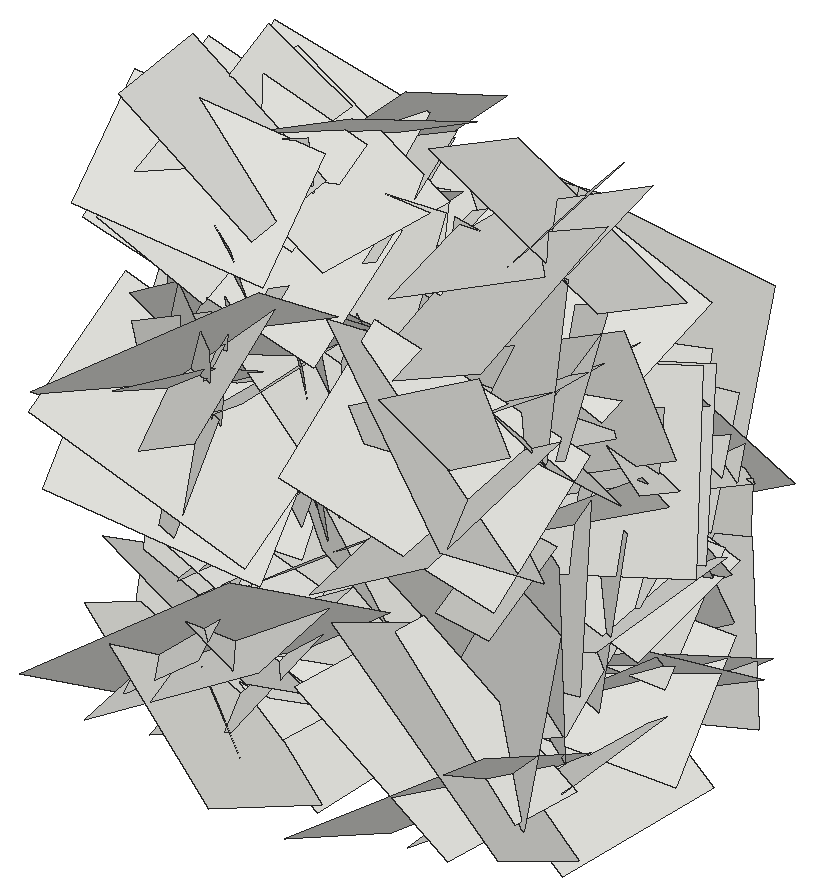
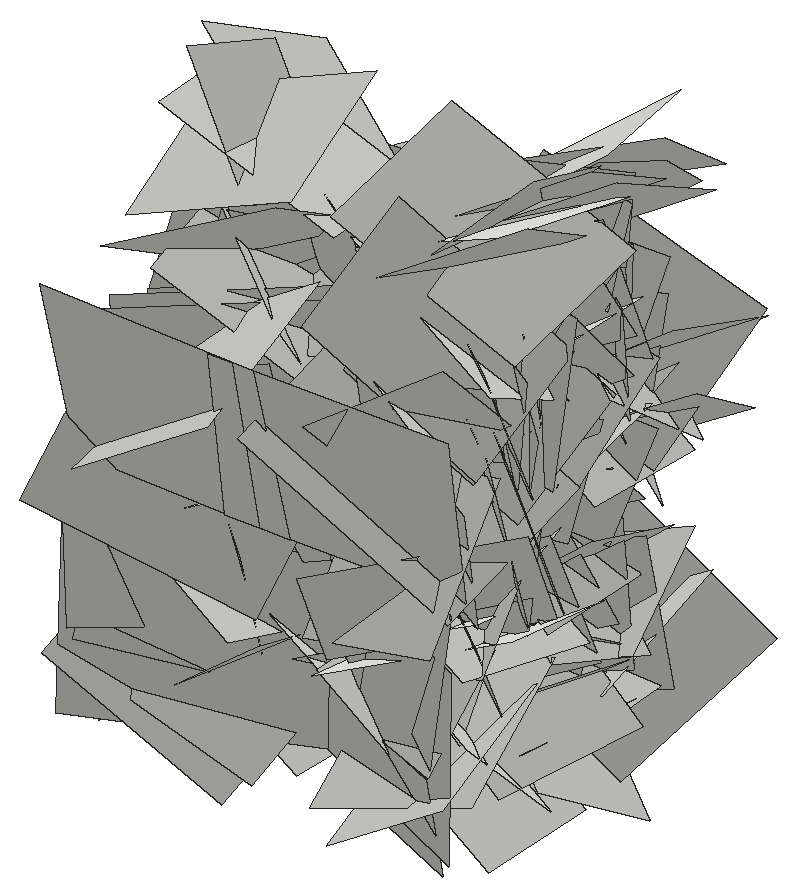
# SketchUp Ruby script. Lengths in inches.
U = 1.inch
M = Sketchup.active_model
def pt(a) = Geom::Point3d.new(a.map { |v| v * U })
def face(e, loops, mat)
  f = e.add_face(loops[0].map { |a| pt(a) })
  loops[1..].each { |l| e.add_face(l.map { |a| pt(a) }).erase! }
  f.material = f.back_material = mat if mat
  f
end
# faces: each face lists its corners as indices into pts; further lists are holes
def faces(e, pts, list, mat = nil) = list.each { |f| face(e, (f[0].is_a?(Array) ? f : [f]).map { |l| l.map { |i| pts[i] } }, mat) }
# xy, xz, yz: faces in a plane at the given z, y or x. An outline is a flat list of corners, or four numbers for a rectangle; further outlines are holes
def ring(l) = l.size == 4 ? [[l[0], l[1]], [l[2], l[1]], [l[2], l[3]], [l[0], l[3]]] : l.each_slice(2).to_a
def flat(e, list, mat, &to3) = list.each { |f| face(e, (f[0].is_a?(Array) ? f : [f]).map { |l| ring(l).map { |u, v| to3.(u, v) } }, mat) }
def xy(e, z, list, mat = nil) = flat(e, list, mat) { |x, y| [x, y, z] }
def xz(e, y, list, mat = nil) = flat(e, list, mat) { |x, z| [x, y, z] }
def yz(e, x, list, mat = nil) = flat(e, list, mat) { |y, z| [x, y, z] }
def lines(e, pts, list) = list.each { |a, b| e.add_line(pt(pts[a]), pt(pts[b])) }
# prism: a flat outline (further loops are holes) pulled along v
def prism(e, loops, v, mat = nil)
  f = face(e, loops, mat); d = Geom::Vector3d.new(v.map { |x| x * U })
  f.pushpull(f.normal.samedirection?(d) ? d.length : -d.length)
end
def box(e, o, s, mat = nil) = prism(e, [[o, [o[0] + s[0], o[1], o[2]], [o[0] + s[0], o[1] + s[1], o[2]], [o[0], o[1] + s[1], o[2]]]], [0, 0, s[2]], mat)
def at(x, y, z, deg = 0) = Geom::Transformation.translation(pt([x, y, z])) * Geom::Transformation.rotation(ORIGIN, Z_AXIS, deg.degrees)
def axes(o, x, y, z) = Geom::Transformation.new([*x, 0, *y, 0, *z, 0, *pt(o).to_a, 1])
def part(name) = M.definitions.add(name)
# library, detail: a bought-in or finely detailed component or shape, given as its bounding box
def library(name, o, s) = part(name).tap { |d| box(d.entities, o, s) }
def detail(e, o, s) = box(e.add_group.entities, o, s)
def put(e, d, t, mat = nil) = e.add_instance(d, t).tap { |i| i.material = mat if mat }
def group(e, t, mat = nil) = e.add_group.tap { |g| g.transformation = t; g.material = mat if mat }.entities
root = M.entities
c1 = part("Component\#6")
p = [[0.01,0,0],[0,3.24,4.54],[4.32,3.24,4.54],[4.33,0,0]]
faces(c1.entities,p,[[0,1,2,3]])
put(root,c1,axes([414.68,209.1,25.86],[0.06992,-0.92649,-0.30548],[0.11921,-0.29692,0.92479],[-1.02719,-0.09753,0.08653]))
put(root,c1,axes([410.71,209.1,25.86],[-0.06992,-0.92649,-0.30548],[-0.11921,-0.29692,0.92479],[1.02719,-0.09753,0.08653]))
put(root,c1,axes([410.71,210.17,27.25],[0.0389,-0.19659,0.74237],[0.03773,0.74285,0.19496],[0.81316,-0.02506,-0.04456]))
put(root,c1,axes([414.68,202.89,32.22],[0.0211,0.0618,0.84202],[0.01452,0.84212,-0.06213],[-0.89482,0.01512,0.01885]))
put(root,c1,axes([410.71,209.27,26.87],[0.02942,-0.98917,0.00062],[-0.2303,-0.00549,0.9654],[1.02292,0.02721,0.21733]))
put(root,c1,axes([410.71,208.86,27.22],[-0.22907,0.58895,0.94038],[-0.09031,0.94642,-0.61231],[1.17269,0.18793,0.13653]))
put(root,c1,axes([410.71,209.72,22.08],[-0.18138,-0.91546,-0.54155],[-0.07402,-0.53767,0.93095],[1.12504,-0.18297,-0.02606]))
put(root,c1,axes([410.71,200.125,30.08],[-0.25415,0.9144,0.59243],[-0.00684,0.60541,-0.93704],[1.1549,0.20481,0.12483]))
put(root,c1,axes([414.68,207.43,34.16],[-0.11276,0.04323,0.70746],[0.03845,0.71477,-0.03823],[-0.75032,0.03013,-0.10828]))
put(root,c1,axes([410.71,204.07,39.0625],[-0.02986,0.79051,0.40956],[0.00815,0.40997,-0.79076],[0.94369,0.02147,0.01979]))
put(root,c1,axes([414.68,209.14,33.82],[-0.16184,0.36707,0.52708],[0.01835,0.54392,-0.37378],[-0.68059,-0.07262,-0.13541]))
put(root,c1,axes([410.71,210.92,34.25],[0.13403,0.53039,0.57824],[-0.04314,0.58935,-0.53168],[0.83061,-0.05497,-0.12092]))
put(root,c1,axes([414.68,209.37,33.75],[0.00852,0.3462,-0.76666],[0.09329,-0.76284,-0.34355],[-0.88678,-0.07692,-0.04351]))
put(root,c1,axes([414.68,201.89,25.36],[-0.12511,0.60489,0.30184],[0.04372,0.31228,-0.60968],[-0.71524,-0.08672,-0.09007]))
put(root,c1,axes([410.71,206.58,28.49],[0.01093,-0.51913,0.63451],[0.10311,0.63085,0.51456],[0.86287,-0.06881,-0.06953]))
put(root,c1,axes([414.68,207.4,37.82],[0.14382,-0.92009,0.02073],[0.06912,0.03051,0.92748],[-0.97309,-0.13382,0.06894]))
put(root,c1,axes([414.68,211.91,37.97],[0.10192,-0.72839,-0.40458],[0.00784,-0.4065,0.73361],[-0.88316,-0.08767,-0.04018]))
put(root,c1,axes([414.68,205,37.54],[-0.1597,-0.46751,-0.41946],[0.05532,-0.43919,0.47075],[-0.66349,0.07592,0.14021]))
put(root,c1,axes([410.71,204.65,32.19],[0.14144,0.68446,-0.34907],[0.03425,-0.35898,-0.69154],[0.81371,-0.10387,0.08978]))
put(root,c1,axes([410.71,205.35,34.65],[0.12302,0.37909,0.72016],[-0.00858,0.72795,-0.38188],[0.86263,-0.04682,-0.1065]))
put(root,c1,axes([414.68,209.27,26.93],[-0.01951,-0.6006,0.29742],[-0.06663,0.29777,0.59742],[-0.70729,-0.01148,-0.06448]))
put(root,c1,axes([414.68,204.33,34.72],[0.02793,-0.28222,0.66343],[-0.05268,0.66158,0.28341],[-0.7624,-0.05605,0.00473]))
put(root,c1,axes([410.71,210.23,35.31],[0.06568,0.00099,-0.81141],[0.08224,-0.81005,0.00494],[0.85616,0.07773,0.06177]))
put(root,c1,axes([414.68,207.11,31.75],[0.23783,0.22127,0.93353],[0.03566,0.95632,-0.23476],[-1.01634,0.08533,0.21022]))
put(root,c1,axes([410.71,201.41,38.375],[-0.12316,0.77538,0.57304],[0.12545,0.58429,-0.76661],[1.01427,0.02189,0.1644]))
put(root,c1,axes([410.71,210.61,30.96],[0.02538,-1.03384,0.49264],[-0.2847,0.47394,1.00764],[1.18007,0.13657,0.23251]))
put(root,c1,axes([410.71,212.48,33.12],[0.02538,-1.03384,0.49264],[-0.2847,0.47394,1.00764],[1.18007,0.13657,0.23251]))
put(root,c1,axes([414.68,206.77,29.69],[-0.13468,0.0618,0.68245],[0.14259,0.68282,-0.03679],[-0.71222,0.12502,-0.13642]))
put(root,c1,axes([410.71,202.75,27.49],[-0.17368,0.85862,-0.51485],[0.1903,-0.48804,-0.87105],[1.04401,0.2318,0.07312]))
put(root,c1,axes([414.68,211.1,35.2],[-0.07899,0.5337,0.27791],[-0.02897,0.27674,-0.53878],[-0.63716,-0.07875,-0.00996]))
put(root,c1,axes([414.68,212.78,35.18],[0.06835,-0.19577,-0.64021],[-0.13077,-0.63563,0.18195],[-0.69749,0.09999,-0.09685]))
put(root,c1,axes([414.68,200.85,29.625],[0.04324,0.39016,0.69087],[0.10275,0.68414,-0.39209],[-0.83473,0.10443,-0.01247]))
put(root,c1,axes([414.68,202.23,33.91],[-0.02493,0.60398,0.49928],[0.17768,0.49182,-0.58706],[-0.81142,0.08914,-0.14389]))
put(root,c1,axes([414.68,204.22,36.67],[-0.08595,0.41822,-0.43473],[0.01861,-0.43682,-0.42351],[-0.63917,-0.06896,0.04613]))
put(root,c1,axes([414.68,206.625,39.5],[0.00312,0.09172,-0.66161],[-0.00201,-0.66161,-0.09173],[-0.70801,0.00228,-0.00265]))
put(root,c1,axes([414.68,212.36,26.625],[0.06935,-0.64087,-0.11796],[-0.11905,-0.12787,0.63241],[-0.68039,-0.04294,-0.12268]))
put(root,c1,axes([414.68,204.95,35.05],[-0.03568,0.1968,-0.61743],[0.04358,-0.61637,-0.1987],[-0.68554,-0.04943,0.01951]))
put(root,c1,axes([410.71,207.21,30.03],[-0.00943,-1.01637,-0.0193],[-0.00822,-0.01923,1.01638],[1.07752,-0.00904,0.00758]))
put(root,c1,axes([410.71,205.67,24.52],[0.15369,0.87531,0.08009],[-0.01982,0.08422,-0.88666],[0.9315,-0.14262,-0.03208]))
put(root,c1,axes([410.71,206.36,33.23],[-0.09168,1.1059,0.20164],[-0.04784,0.19866,-1.1089],[1.19063,0.09314,-0.02903]))
put(root,c1,axes([410.71,211.47,22.62],[-0.20513,-1.22241,0.07319],[-0.04122,0.08019,1.23659],[1.29742,-0.19072,0.05085]))
put(root,c1,axes([414.68,202.42,34.22],[0.03507,0.56649,-0.26791],[-0.06705,-0.26389,-0.56581],[-0.66085,0.05684,0.04319]))
put(root,c1,axes([414.68,203.96,20.97],[-0.02025,-0.24988,0.58047],[0.03388,0.57961,0.25056],[-0.66903,0.03691,-0.00488]))
put(root,c1,axes([414.68,208.95,27.68],[0.1117,0.11156,-0.75397],[0.06454,-0.75994,-0.10393],[-0.80532,-0.04543,-0.11291]))
put(root,c1,axes([414.68,211.4,20.36],[0.11841,0.02386,0.67628],[-0.07272,0.6823,-0.01274],[-0.7136,-0.06557,0.11352]))
put(root,c1,axes([410.71,209.77,25.57],[-0.04769,1.02209,-0.46416],[-0.05126,-0.46587,-1.02116],[1.18879,0.02092,-0.06265]))
put(root,c1,axes([410.71,212.41,27.7],[0.11035,-0.46639,-0.85158],[-0.0233,-0.85737,0.46687],[1.02892,0.03061,0.1019]))
put(root,c1,axes([414.68,210.37,37.54],[0.0852,-0.7988,-0.26142],[0.21653,-0.23617,0.78446],[-0.8642,-0.13792,0.17078]))
put(root,c1,axes([414.68,207.84,29.22],[0.13906,-0.51177,-0.49755],[-0.00544,-0.50655,0.51967],[-0.75658,-0.09042,-0.09518]))
put(root,c1,axes([410.71,211.63,27.44],[0.13698,0.50835,-0.7639],[0.02564,-0.77306,-0.51036],[0.97231,-0.05123,0.12108]))
put(root,c1,axes([410.71,212.85,24.81],[-0.10314,-0.72888,-0.73382],[0.20394,-0.73695,0.70648],[1.07722,0.06973,-0.20401]))
put(root,c1,axes([410.71,211.43,33.78],[-0.23599,-0.36182,-1.29322],[-0.09706,-1.30373,0.38052],[1.42014,-0.14923,-0.18889]))
put(root,c1,axes([410.71,199.54,32.72],[-0.14681,1.15124,0.44909],[-0.05729,0.44582,-1.15954],[1.30862,0.14867,-0.00039]))
put(root,c1,axes([410.71,206.07,20.81],[-0.31441,-1.20333,0.63493],[-0.01893,0.65323,1.22967],[1.44208,-0.25378,0.15457]))
put(root,c1,axes([410.71,208.01,36.375],[-0.10923,0.38133,-1.06486],[0.05778,-1.06635,-0.38714],[1.19755,0.08623,-0.07845]))
put(root,c1,axes([410.71,212.99,32.26],[0.05541,-0.21084,-0.92918],[0.15034,-0.91849,0.21639],[0.99872,0.14996,0.01898]))
put(root,c1,axes([410.71,205.46,33.43],[0.14097,0.63084,0.7943],[-0.06243,0.80455,-0.62912],[1.07339,-0.03606,-0.14091]))
put(root,c1,axes([410.71,207.91,30.98],[-0.03881,-0.77727,0.6188],[0.26695,0.59174,0.75817],[1.01873,-0.18467,-0.1751]))
put(root,c1,axes([414.68,206,31.6],[0.1462,-0.08624,0.716],[0.07336,0.72719,0.07426],[-0.76092,0.05354,0.14472]))
put(root,c1,axes([414.68,210.56,30.82],[0.08988,0.23539,0.56706],[-0.00516,0.57268,-0.23699],[-0.65079,0.02797,0.0802]))
put(root,c1,axes([410.71,206.55,33.15],[0.00164,-0.95203,-0.71322],[-0.09471,-0.7113,0.94927],[1.25737,-0.05234,0.07244]))
put(root,c1,axes([410.71,206.8125,26.89],[-0.15204,1.11982,0.24611],[0.19339,0.26716,-1.10927],[1.19986,0.09884,0.20998]))
put(root,c1,axes([410.71,211.99,33.59],[-0.13241,-0.25962,-1.28668],[-0.09489,-1.2878,0.26854],[1.38813,-0.1128,-0.10438]))
put(root,c1,axes([410.71,206.95,24.98],[0.09414,0.39654,1.07266],[-0.12922,1.07305,-0.38659],[1.20532,0.08407,-0.12522]))
put(root,c1,axes([414.68,202.49,32.61],[0.11645,-0.17214,0.59947],[0.01233,0.60916,0.17278],[-0.661,-0.01896,0.10883]))
put(root,c1,axes([410.71,205.38,23.16],[0.04798,1.09948,0.05597],[0.01409,0.05547,-1.10036],[1.16688,-0.04588,0.01099]))
put(root,c1,axes([410.71,210.75,36.02],[-0.14272,-1.0645,0.43866],[0.22696,0.41079,1.0626],[1.19913,-0.20445,-0.14891]))
put(root,c1,axes([410.71,208.81,31.45],[-0.04602,0.84125,-1.04893],[-0.18208,-1.04435,-0.83047],[1.4136,-0.10713,-0.14111]))
put(root,c1,axes([410.71,213.59,29.33],[0.10669,0.07311,-1.12569],[-0.06812,-1.12796,-0.079],[1.19381,-0.0709,0.09609]))
put(root,c1,axes([410.71,201.95,25.76],[0.02109,1.10253,-0.4508],[-0.04504,-0.44992,-1.10225],[1.2618,-0.03449,-0.03181]))
put(root,c1,axes([410.71,213.06,27.02],[-0.109,-1.16412,-0.17966],[0.1638,-0.19212,1.15639],[1.23778,-0.07709,-0.16885]))
put(root,c1,axes([410.71,201.85,37.73],[-0.10519,1.13817,0.58904],[-0.00109,0.59073,-1.14161],[1.35845,0.08861,0.0447]))
put(root,c1,axes([410.71,204.59,30.02],[-0.04301,-1.09683,0.72238],[-0.12053,0.72294,1.0913],[1.38692,0.02882,0.11724]))
put(root,c1,axes([410.71,209.74,33.23],[0.15201,0.07034,-1.21602],[-0.20156,-1.20811,-0.09231],[1.2753,-0.19933,0.13035]))
put(root,c1,axes([410.71,208.94,26.04],[-0.1299,1.02121,-0.60997],[0.25035,-0.5801,-1.01865],[1.23578,0.22487,0.14225]))
put(root,c1,axes([410.71,213.71,29.11],[-0.07729,-1.24842,0.49404],[-0.03127,0.49613,1.24937],[1.42283,-0.05691,0.0543]))
put(root,c1,axes([410.71,211.375,32.78],[-0.08242,0.8278,-0.94283],[0.12426,-0.93571,-0.83122],[1.32412,0.13934,0.01932]))
put(root,c1,axes([410.71,211.85,35.53],[0.11979,-0.95717,-0.48165],[0.13908,-0.46832,0.96146],[1.12727,0.15949,-0.06744]))
put(root,c1,axes([410.71,203.71,22.72],[-0.0324,0.32539,1.27516],[0.00551,1.27553,-0.32536],[1.39498,0.00251,0.0309]))
put(root,c1,axes([410.71,205.99,22.98],[0.14358,-1.11124,-0.06865],[0.09474,-0.05808,1.11649],[1.17635,0.14031,-0.08154]))
put(root,c1,axes([410.71,205.63,39.17],[0.17317,1.06099,0.10432],[0.22006,0.07185,-1.05594],[1.10844,-0.18002,0.19334]))
put(root,c1,axes([410.71,205.46,24.09],[0.08024,0.04196,1.34674],[-0.06239,1.34768,-0.03868],[1.42687,0.05657,-0.07742]))
put(root,c1,axes([410.71,204.65,33.57],[0.11682,0.36237,1.1463],[0.15256,1.13885,-0.37385],[1.26518,-0.17079,-0.06076]))
put(root,c1,axes([410.71,211.92,20.51],[0.20622,-1.25394,-0.15944],[-0.06822,-0.17093,1.26581],[1.33814,0.18453,0.0891]))
put(root,c1,axes([410.71,213.57,27.56],[-0.01798,0.03957,-1.39555],[0.22262,-1.3797,-0.04168],[1.46303,0.21042,-0.01081]))
put(root,c1,axes([410.71,205.51,24.88],[0.13882,1.11155,0.63897],[0.19603,0.6192,-1.11507],[1.34484,-0.205,0.09658]))
put(root,c1,axes([410.37,214.11,35.21],[0.07772,-0.27644,-1.33377],[0.91911,-1.02064,0.2592],[1.11351,0.86175,-0.12086]))
put(root,c1,axes([410.71,205.05,35.75],[0.23328,1.34713,-0.22992],[0.05022,-0.24027,-1.36238],[1.44774,-0.20874,0.08431]))
put(root,c1,axes([410.71,206.12,25.83],[0.28838,0.48251,1.20317],[0.13396,1.21365,-0.51529],[1.36755,-0.22063,-0.20324]))
put(root,c1,axes([424.49,206.12,25.83],[-0.28838,0.48251,1.20317],[-0.13396,1.21365,-0.51529],[-1.36755,-0.22063,-0.20324]))
put(root,c1,axes([424.49,205.05,35.75],[-0.23328,1.34713,-0.22992],[-0.05022,-0.24027,-1.36238],[-1.44774,-0.20874,0.08431]))
put(root,c1,axes([424.83,214.11,35.21],[-0.07772,-0.27644,-1.33377],[-0.91911,-1.02064,0.2592],[-1.11351,0.86175,-0.12086]))
put(root,c1,axes([424.49,205.51,24.88],[-0.13882,1.11155,0.63897],[-0.19603,0.6192,-1.11507],[-1.34484,-0.205,0.09658]))
put(root,c1,axes([424.49,213.57,27.56],[0.01798,0.03957,-1.39555],[-0.22262,-1.3797,-0.04168],[-1.46303,0.21042,-0.01081]))
put(root,c1,axes([424.49,211.92,20.51],[-0.20622,-1.25394,-0.15944],[0.06822,-0.17093,1.26581],[-1.33814,0.18453,0.0891]))
put(root,c1,axes([424.49,204.65,33.57],[-0.11682,0.36237,1.1463],[-0.15256,1.13885,-0.37385],[-1.26518,-0.17079,-0.06076]))
put(root,c1,axes([424.49,205.46,24.09],[-0.08024,0.04196,1.34674],[0.06239,1.34768,-0.03868],[-1.42687,0.05657,-0.07742]))
put(root,c1,axes([424.49,205.63,39.17],[-0.17317,1.06099,0.10432],[-0.22006,0.07185,-1.05594],[-1.10844,-0.18002,0.19334]))
put(root,c1,axes([424.49,205.99,22.98],[-0.14358,-1.11124,-0.06865],[-0.09474,-0.05808,1.11649],[-1.17635,0.14031,-0.08154]))
put(root,c1,axes([424.49,203.71,22.72],[0.0324,0.32539,1.27516],[-0.00551,1.27553,-0.32536],[-1.39498,0.00251,0.0309]))
put(root,c1,axes([424.49,211.85,35.53],[-0.11979,-0.95717,-0.48165],[-0.13908,-0.46832,0.96146],[-1.12727,0.15949,-0.06744]))
put(root,c1,axes([424.49,211.375,32.78],[0.08242,0.8278,-0.94283],[-0.12426,-0.93571,-0.83122],[-1.32412,0.13934,0.01932]))
put(root,c1,axes([424.49,213.71,29.11],[0.07729,-1.24842,0.49404],[0.03127,0.49613,1.24937],[-1.42283,-0.05691,0.0543]))
put(root,c1,axes([424.49,208.94,26.04],[0.1299,1.02121,-0.60997],[-0.25035,-0.5801,-1.01865],[-1.23578,0.22487,0.14225]))
put(root,c1,axes([424.49,209.74,33.23],[-0.15201,0.07034,-1.21602],[0.20156,-1.20811,-0.09231],[-1.2753,-0.19933,0.13035]))
put(root,c1,axes([424.49,204.59,30.02],[0.04301,-1.09683,0.72238],[0.12053,0.72294,1.0913],[-1.38692,0.02882,0.11724]))
put(root,c1,axes([424.49,201.85,37.73],[0.10519,1.13817,0.58904],[0.00109,0.59073,-1.14161],[-1.35845,0.08861,0.0447]))
put(root,c1,axes([424.49,213.06,27.02],[0.109,-1.16412,-0.17966],[-0.1638,-0.19212,1.15639],[-1.23778,-0.07709,-0.16885]))
put(root,c1,axes([424.49,201.95,25.76],[-0.02109,1.10253,-0.4508],[0.04504,-0.44992,-1.10225],[-1.2618,-0.03449,-0.03181]))
put(root,c1,axes([424.49,213.59,29.33],[-0.10669,0.07311,-1.12569],[0.06812,-1.12796,-0.079],[-1.19381,-0.0709,0.09609]))
put(root,c1,axes([424.49,208.81,31.45],[0.04602,0.84125,-1.04893],[0.18208,-1.04435,-0.83047],[-1.4136,-0.10713,-0.14111]))
put(root,c1,axes([424.49,210.75,36.02],[0.14272,-1.0645,0.43866],[-0.22696,0.41079,1.0626],[-1.19913,-0.20445,-0.14891]))
put(root,c1,axes([424.49,205.38,23.16],[-0.04798,1.09948,0.05597],[-0.01409,0.05547,-1.10036],[-1.16688,-0.04588,0.01099]))
put(root,c1,axes([420.52,202.49,32.61],[-0.11645,-0.17214,0.59947],[-0.01233,0.60916,0.17278],[0.661,-0.01896,0.10883]))
put(root,c1,axes([424.49,206.95,24.98],[-0.09414,0.39654,1.07266],[0.12922,1.07305,-0.38659],[-1.20532,0.08407,-0.12522]))
put(root,c1,axes([424.49,211.99,33.59],[0.13241,-0.25962,-1.28668],[0.09489,-1.2878,0.26854],[-1.38813,-0.1128,-0.10438]))
put(root,c1,axes([424.49,206.8125,26.89],[0.15204,1.11982,0.24611],[-0.19339,0.26716,-1.10927],[-1.19986,0.09884,0.20998]))
put(root,c1,axes([424.49,206.55,33.15],[-0.00164,-0.95203,-0.71322],[0.09471,-0.7113,0.94927],[-1.25737,-0.05234,0.07244]))
put(root,c1,axes([420.52,210.56,30.82],[-0.08988,0.23539,0.56706],[0.00516,0.57268,-0.23699],[0.65079,0.02797,0.0802]))
put(root,c1,axes([420.52,206,31.6],[-0.1462,-0.08624,0.716],[-0.07336,0.72719,0.07426],[0.76092,0.05354,0.14472]))
put(root,c1,axes([424.49,207.91,30.98],[0.03881,-0.77727,0.6188],[-0.26695,0.59174,0.75817],[-1.01873,-0.18467,-0.1751]))
put(root,c1,axes([424.49,205.46,33.43],[-0.14097,0.63084,0.7943],[0.06243,0.80455,-0.62912],[-1.07339,-0.03606,-0.14091]))
put(root,c1,axes([424.49,212.99,32.26],[-0.05541,-0.21084,-0.92918],[-0.15034,-0.91849,0.21639],[-0.99872,0.14996,0.01898]))
put(root,c1,axes([424.49,208.01,36.375],[0.10923,0.38133,-1.06486],[-0.05778,-1.06635,-0.38714],[-1.19755,0.08623,-0.07845]))
put(root,c1,axes([424.49,206.07,20.81],[0.31441,-1.20333,0.63493],[0.01893,0.65323,1.22967],[-1.44208,-0.25378,0.15457]))
put(root,c1,axes([424.49,199.54,32.72],[0.14681,1.15124,0.44909],[0.05729,0.44582,-1.15954],[-1.30862,0.14867,-0.00039]))
put(root,c1,axes([424.49,211.43,33.78],[0.23599,-0.36182,-1.29322],[0.09706,-1.30373,0.38052],[-1.42014,-0.14923,-0.18889]))
put(root,c1,axes([424.49,212.85,24.81],[0.10314,-0.72888,-0.73382],[-0.20394,-0.73695,0.70648],[-1.07722,0.06973,-0.20401]))
put(root,c1,axes([424.49,211.63,27.44],[-0.13698,0.50835,-0.7639],[-0.02564,-0.77306,-0.51036],[-0.97231,-0.05123,0.12108]))
put(root,c1,axes([420.52,207.84,29.22],[-0.13906,-0.51177,-0.49755],[0.00544,-0.50655,0.51967],[0.75658,-0.09042,-0.09518]))
put(root,c1,axes([420.52,210.37,37.54],[-0.0852,-0.7988,-0.26142],[-0.21653,-0.23617,0.78446],[0.8642,-0.13792,0.17078]))
put(root,c1,axes([424.49,212.41,27.7],[-0.11035,-0.46639,-0.85158],[0.0233,-0.85737,0.46687],[-1.02892,0.03061,0.1019]))
put(root,c1,axes([424.49,209.77,25.57],[0.04769,1.02209,-0.46416],[0.05126,-0.46587,-1.02116],[-1.18879,0.02092,-0.06265]))
